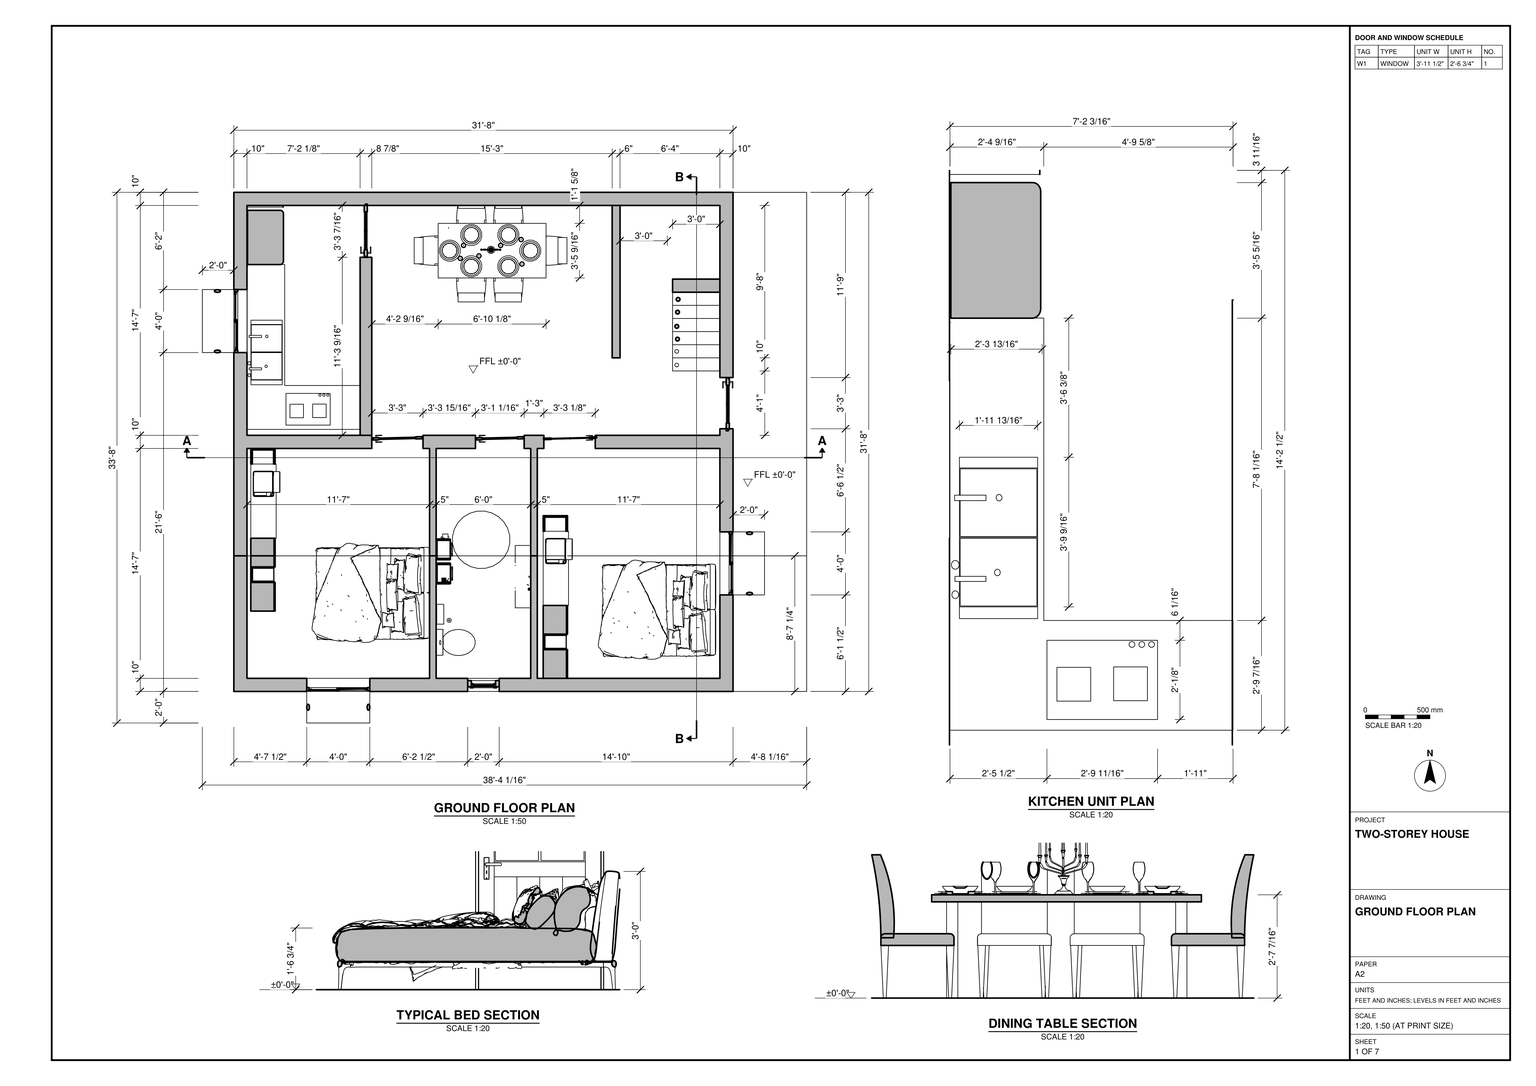
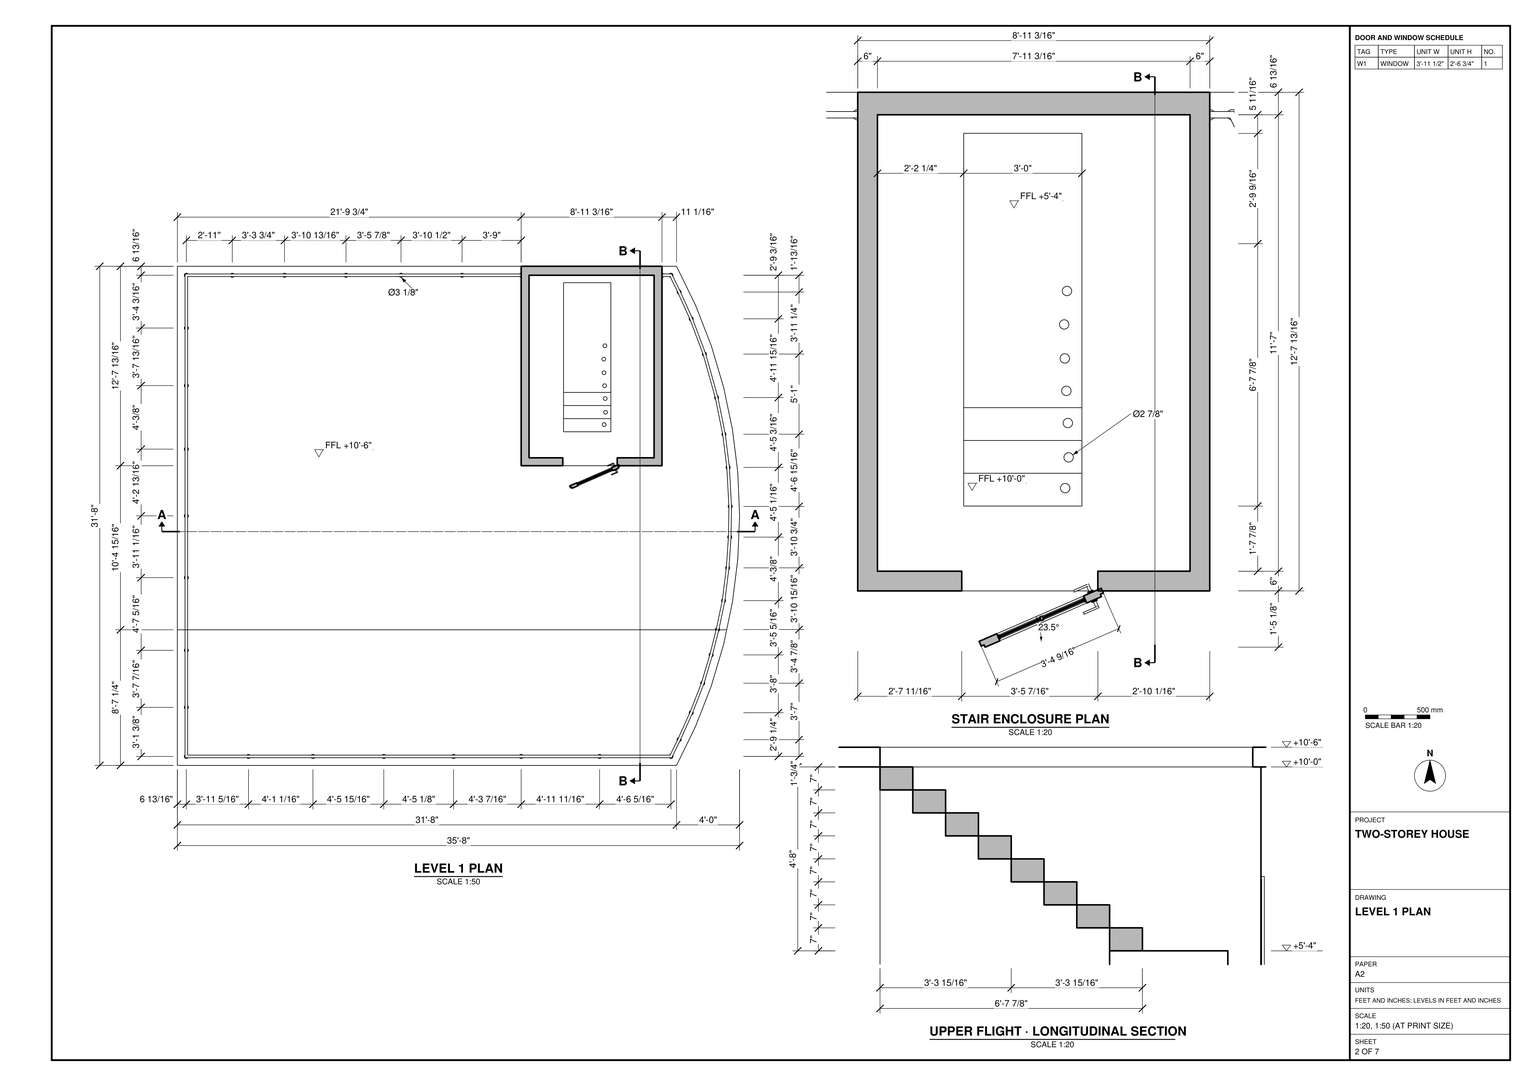
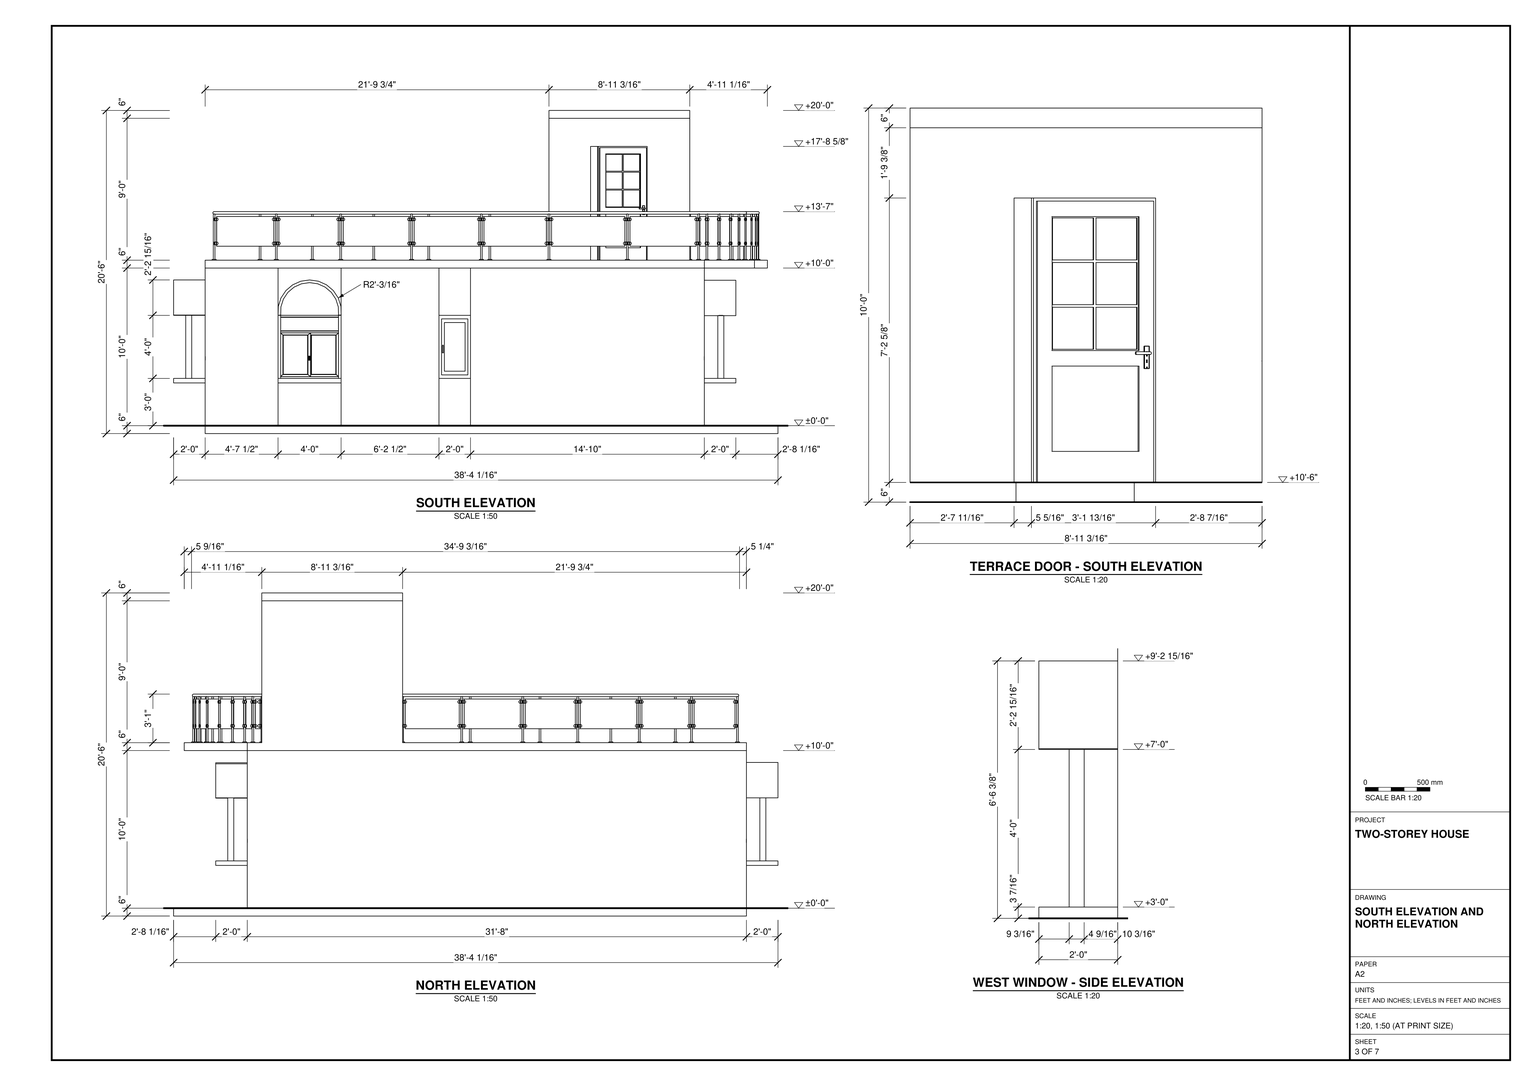
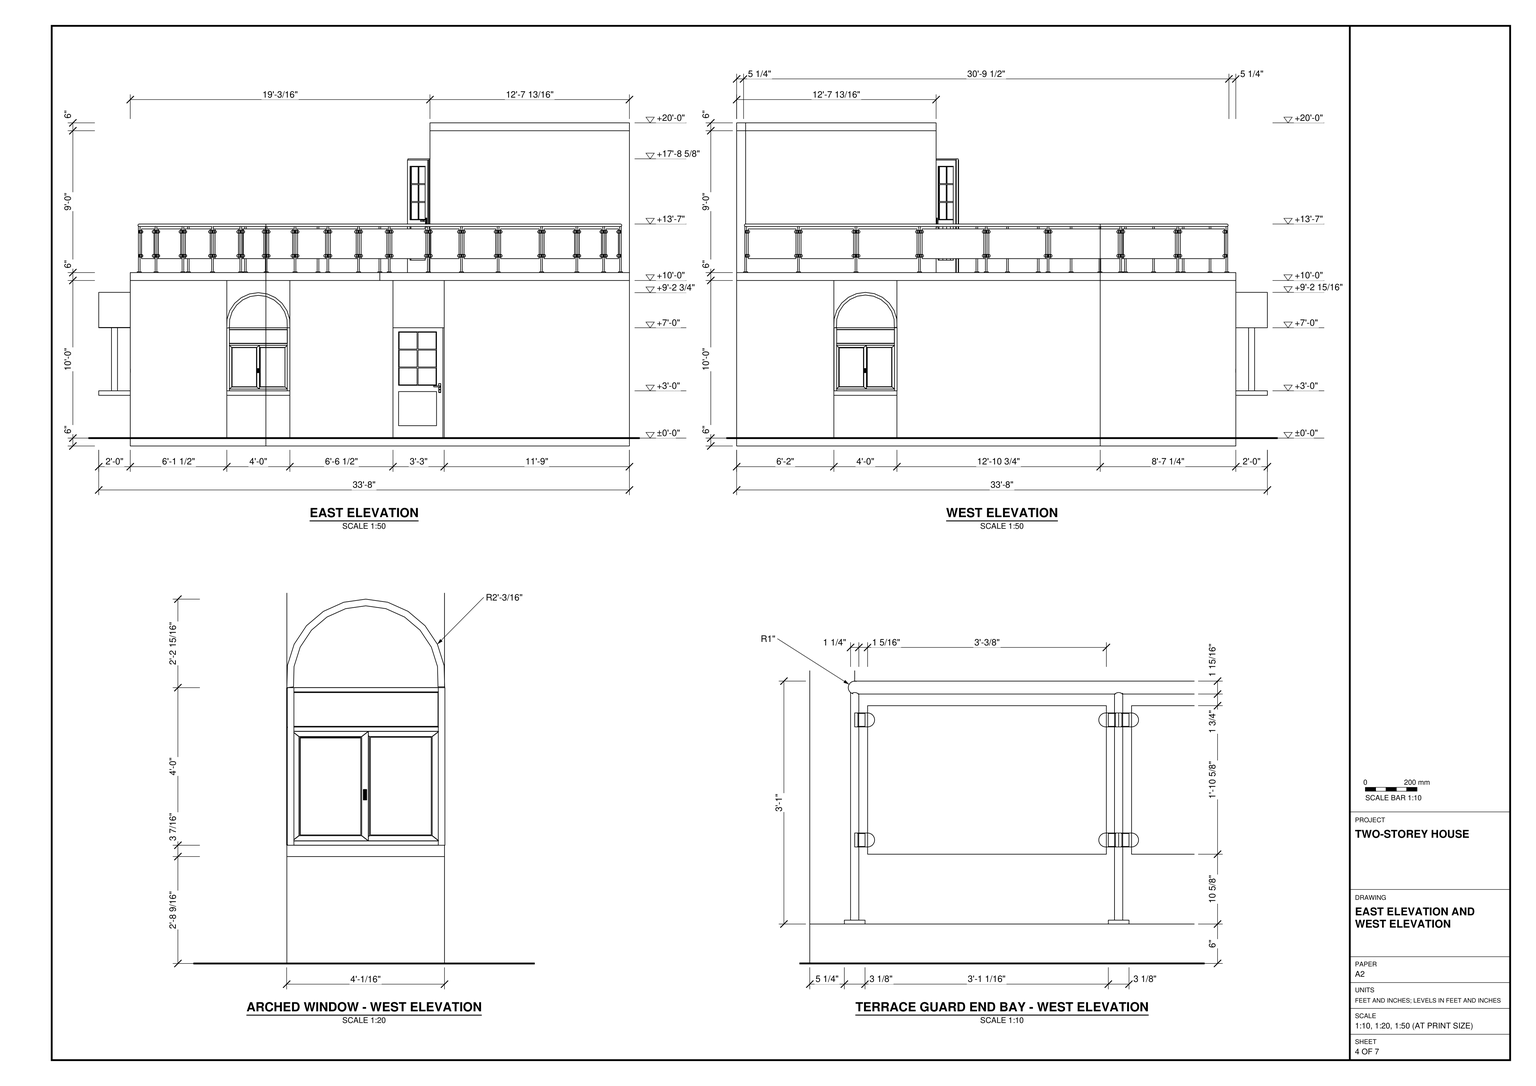
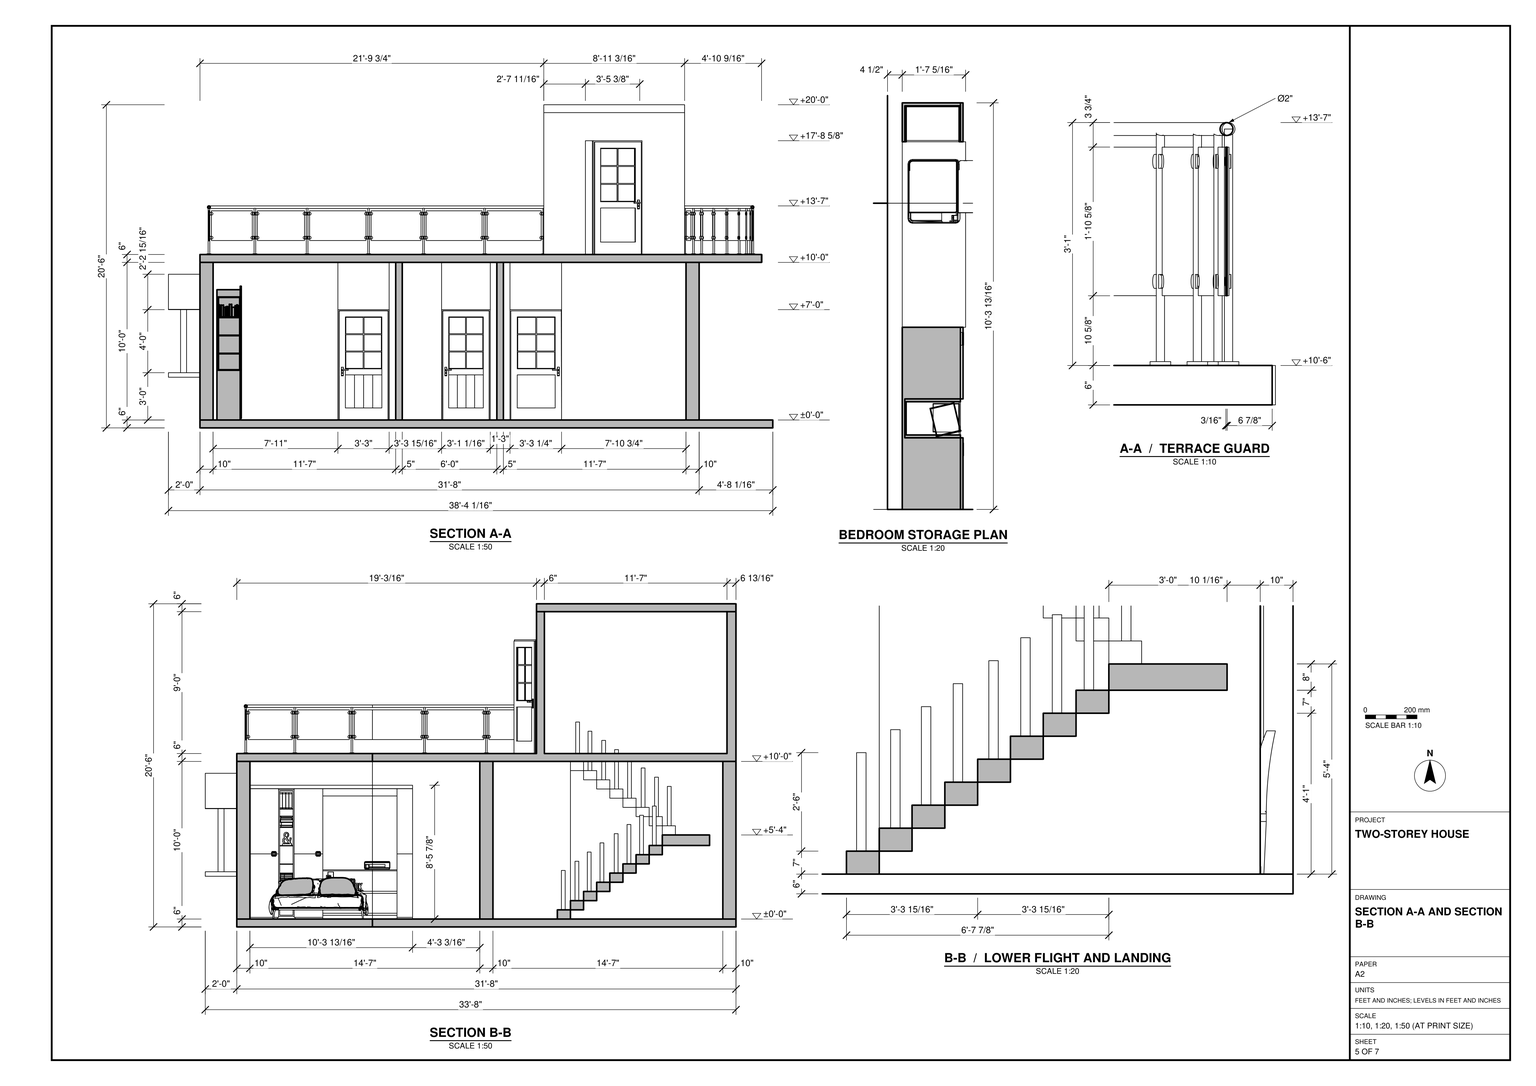
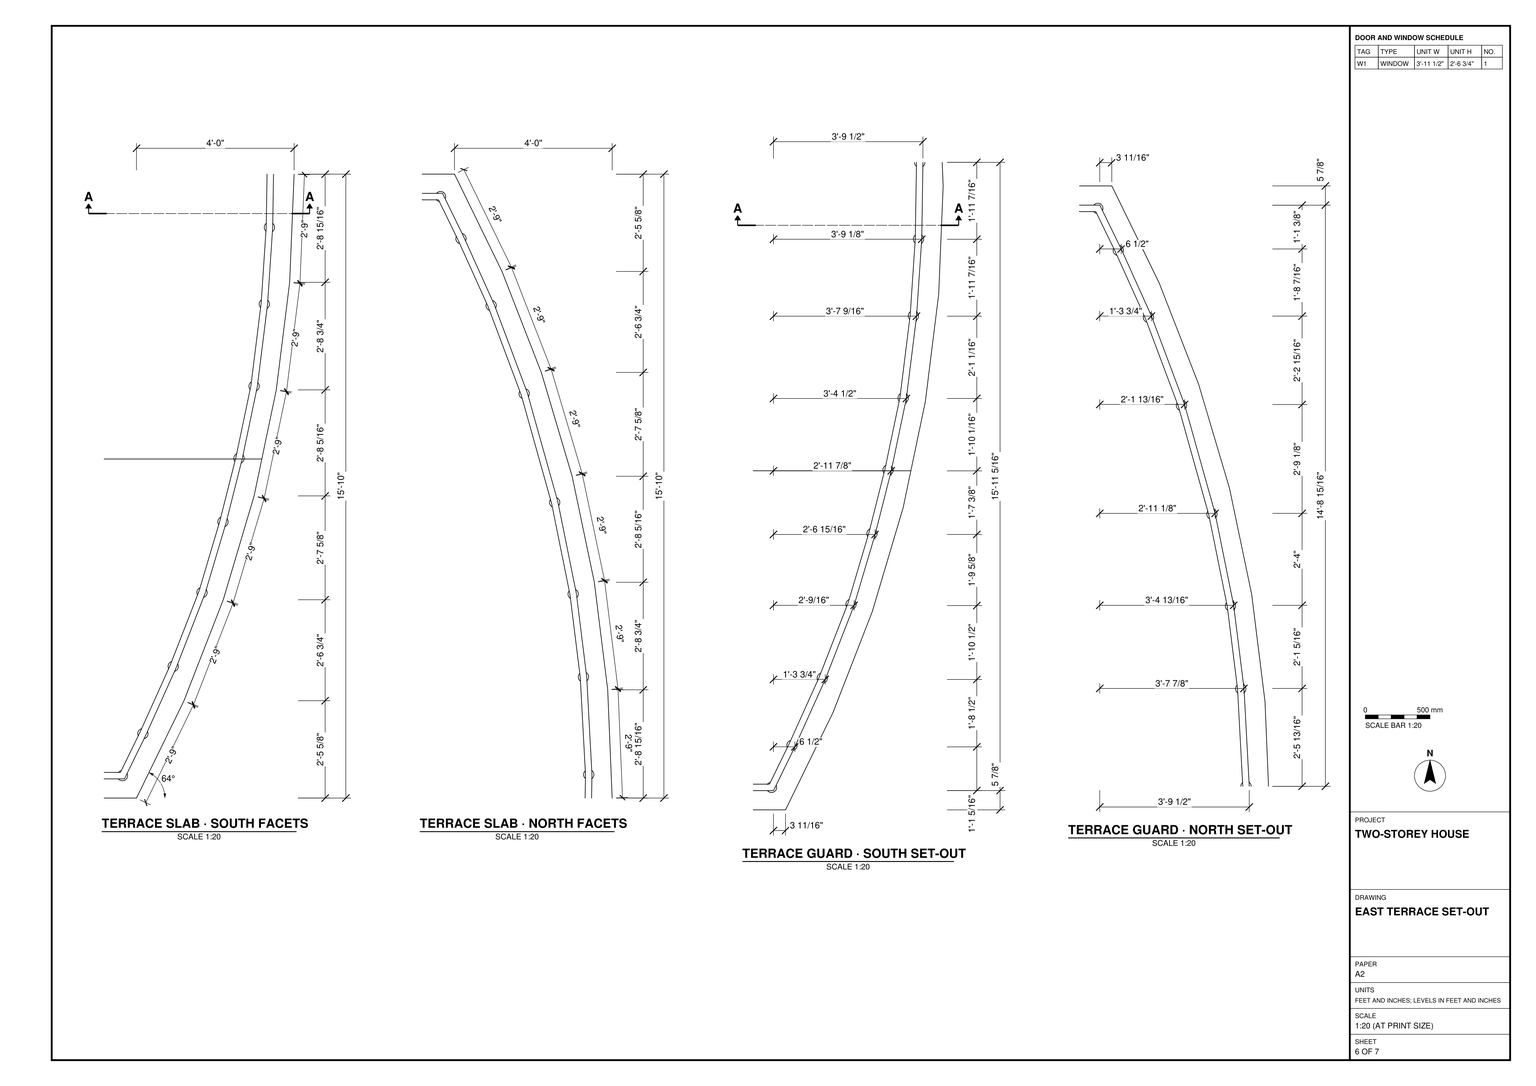
Build the house in SketchUp from task_files/diagram_01.pdf. Work in feet and inches. The overall model extents, including projections, are 38'-4 1/16" east to west, 33'-8" north to south and 20'-6" vertically. Set the ground floor at ±0'-0" and the upper level at +10'-0". Distinguish the upper level from the terrace surface at +10'-6".

Model the ground slab, exterior walls and internal partitions with the thicknesses shown in plan. Place the two bedrooms along the south wall with the bathroom between them. Fit out the bedrooms with the beds and wall-side furniture shown. Place the L-shaped kitchen in the northwest corner, the dining table and chairs beside it, and the stair to the northeast. Form the door and window openings in their drawn positions, including the projecting window heads and sills shown in elevation.

Connect the stair flights at the intermediate landing. Above them, model the flat-roofed stair enclosure and its glazed door onto the terrace. Follow the curved east edge of the terrace slab in plan and carry the railing around the exposed perimeter. Decor and loose items may be any suitable library components.

Keep shell elements such as walls, slabs and roofs, and each furniture or joinery piece, in separate groups or components. Use components for repeated parts. Save one SketchUp model as output_files/two_storey_house_with_a_curved_edge_roof_terrace.skp.

# SketchUp Ruby script. Lengths in inches.
U = 1.inch
M = Sketchup.active_model
def pt(a) = Geom::Point3d.new(a.map { |v| v * U })
def face(e, loops, mat)
  f = e.add_face(loops[0].map { |a| pt(a) })
  loops[1..].each { |l| e.add_face(l.map { |a| pt(a) }).erase! }
  f.material = f.back_material = mat if mat
  f
end
# faces: each face lists its corners as indices into pts; further lists are holes
def faces(e, pts, list, mat = nil) = list.each { |f| face(e, (f[0].is_a?(Array) ? f : [f]).map { |l| l.map { |i| pts[i] } }, mat) }
# xy, xz, yz: faces in a plane at the given z, y or x. An outline is a flat list of corners, or four numbers for a rectangle; further outlines are holes
def ring(l) = l.size == 4 ? [[l[0], l[1]], [l[2], l[1]], [l[2], l[3]], [l[0], l[3]]] : l.each_slice(2).to_a
def flat(e, list, mat, &to3) = list.each { |f| face(e, (f[0].is_a?(Array) ? f : [f]).map { |l| ring(l).map { |u, v| to3.(u, v) } }, mat) }
def xy(e, z, list, mat = nil) = flat(e, list, mat) { |x, y| [x, y, z] }
def xz(e, y, list, mat = nil) = flat(e, list, mat) { |x, z| [x, y, z] }
def yz(e, x, list, mat = nil) = flat(e, list, mat) { |y, z| [x, y, z] }
def lines(e, pts, list) = list.each { |a, b| e.add_line(pt(pts[a]), pt(pts[b])) }
# prism: a flat outline (further loops are holes) pulled along v
def prism(e, loops, v, mat = nil)
  f = face(e, loops, mat); d = Geom::Vector3d.new(v.map { |x| x * U })
  f.pushpull(f.normal.samedirection?(d) ? d.length : -d.length)
end
def box(e, o, s, mat = nil) = prism(e, [[o, [o[0] + s[0], o[1], o[2]], [o[0] + s[0], o[1] + s[1], o[2]], [o[0], o[1] + s[1], o[2]]]], [0, 0, s[2]], mat)
def at(x, y, z, deg = 0) = Geom::Transformation.translation(pt([x, y, z])) * Geom::Transformation.rotation(ORIGIN, Z_AXIS, deg.degrees)
def axes(o, x, y, z) = Geom::Transformation.new([*x, 0, *y, 0, *z, 0, *pt(o).to_a, 1])
def part(name) = M.definitions.add(name)
# library, detail: a bought-in or finely detailed component or shape, given as its bounding box
def library(name, o, s) = part(name).tap { |d| box(d.entities, o, s) }
def detail(e, o, s) = box(e.add_group.entities, o, s)
def put(e, d, t, mat = nil) = e.add_instance(d, t).tap { |i| i.material = mat if mat }
def group(e, t, mat = nil) = e.add_group.tap { |g| g.transformation = t; g.material = mat if mat }.entities
root = M.entities
M.materials.add("Material \#26").color = [4, 4, 4]
M.materials.add("Material \#575").color = [127, 127, 127]
M.materials.add("[Color D02]").color = [255, 229, 153]
M.materials.add("[Color D03]").color = [255, 216, 101]
M.materials.add("[Color E02]").color = [255, 255, 153]
M.materials.add("[Color F02]").color = [204, 255, 153]
M.materials.add("[Color I01]").color = [204, 204, 255]
M.materials.add("[Color_000]").color = [255, 255, 255]
M.materials.add("[Color_004]").color = [142, 142, 142]
M.materials.add("[Color_005]").color = [114, 114, 114]
M.materials.add("[Color_007]").color = [58, 58, 58]
M.materials.add("[Translucent Glass Blue]").color = [100, 149, 237]
M.materials["[Translucent Glass Blue]"].alpha = 0.5
M.materials.add("[Translucent Glass Gray]").color = [0, 0, 0]
M.materials["[Translucent Glass Gray]"].alpha = 0.1
M.materials.add("[Wood_ Floor]").color = [155, 105, 61]
M.materials.add("[Wood_Lumber_ButtJoined]").color = [69, 62, 43]
c1 = library("ear swab",[42.94,49.125,-0.01],[11.74,6.52,7.19])
c2 = library("Window with transom",[0,0,0],[5.2,55.12,70.87])
c3 = library("Deur met glas",[0,0,0],[39.37,7.97,86.61])
c4 = library("Composant\#42",[0,0,0],[23.62,8.27,35.43])
c5 = library("Untitled",[0,-0.39,0],[231.1,401.96,270.47])
c6 = library("Dining Table",[54.55,57.53,0],[71.62,106.71,46.43])
c7 = library("Group\#16",[0,0,0],[13.47,43.07,1.47])
c8 = library("Group\#63",[0,0,0],[5.65,13.74,2.92])
c9 = library("Group\#64",[0,0,0],[6.09,14.19,2.01])
c10 = library("Group\#65",[0,0,0],[2.54,2.54,11.95])
c11 = library("Group\#66",[0,0,0],[2.54,2.54,11.95])
c12 = library("Group\#50",[0,0,0],[19.72,19.72,56.95])
c13 = library("Group\#81",[0,0,0],[3.17,3.17,3.01])
c14 = library("Group\#51",[0,0,-141.09],[175,104.42,354])
c15 = library("Group\#99",[0,0,0],[24,48.09,26.96])
c16 = part("Group\#100")
box(c16.entities,[0,0,0],[48,24,3.44])
c17 = part("Group\#3")
box(c17.entities,[0,0,0],[36,9.99,7])
c18 = library("Group\#104",[0,0,0],[2.875,2.875,30])
c19 = library("Group\#105",[0,0,0],[417.17,369.47,36.98])
c20 = part("Group255\#1")
xz(c20.entities,1200.29,[[724.9375,120,1143.1,126]])
c21 = part("Group259\#1")
xz(c21.entities,1200.29,[[724.9375,0,734.9375,120],[873.9375,0,878.9375,120],[950.9375,0,955.9375,120],[1094.9375,0,1104.9375,36],[1094.9375,84,1104.9375,120]],"[Color E02]")
c22 = part("Group261\#1")
xz(c22.entities,1200.29,[[724.9375,-6,1161,0]],"[Color D03]")
c23 = part("Group2139\#1")
xz(c23.entities,1200.29,[[886.94,28.92,887.95,35.86]])
c24 = part("Group2175\#1")
xz(c24.entities,1200.29,[[889.71,0,890.1,28.92]],"[Wood_Lumber_ButtJoined]")
c25 = part("Group2179\#1")
xz(c25.entities,1200.29,[[890.79,25.29,891.39,26.55]],"[Color_005]")
c26 = part("Group2225\#1")
xz(c26.entities,1200.29,[[895.16,-0.23,931.33,0]])
c27 = part("Group2241\#1")
xz(c27.entities,1200.29,[[755.57,49.61,756.36,99.21]],"[Color_007]")
c28 = part("Group2251\#1")
xz(c28.entities,1200.29,[[755.57,1.26,756.36,49.61]],"[Color_007]")
c29 = part("Group2447\#1")
xz(c29.entities,1200.29,[[737.85,0,755.57,99.21]],"[Color_007]")
c30 = part("Group2455\#1")
xz(c30.entities,1200.29,[[755.57,99.29,756.36,101.87]],"[Color_000]")
c31 = part("Group2495\#1")
xz(c31.entities,1200.29,[[978.15,93.7,978.93,99.21]],"[Color_007]")
c32 = part("Group2681\#1")
xz(c32.entities,1200.29,[[960.43,0,960.43,36.69,962.16,36.69,962.16,21.14,978.15,21.14,978.15,19.57,962.16,19.57,962.16,4.41,978.15,4.41,978.15,2.83,962.16,2.83,962.16,0],[960.43,93.7,978.15,99.21]],"[Color_007]")
c33 = part("Group2683\#1")
xz(c33.entities,1200.29,[[963.06,38.07,962.83,38.1,962.42,38.34,962.18,38.74,962.15,38.98,962.15,42.95,962.18,43.1875,962.34,43.46,965.76,43.46,965.76,43.43,974.03,43.43,974.03,43.46,976.85,43.46,977.14,43.39,977.36,43.17,977.4375,42.875,977.4375,41.61,977.04,39.84,969.5,39.84,969.5,38.07],[969.5,38.07,969.52,39.84],[965.76,43.43,974.03,43.44],[962.3125,43.46,962.3125,43.62,962.32,43.68,962.38,43.79,962.49,43.85,962.55,43.86,976.89,43.86,976.95,43.85,977.05,43.79,977.11,43.68,977.12,43.62,977.12,43.46]],"[Color_000]")
c34 = part("Group2685\#1")
xz(c34.entities,1200.29,[[962.86,37.48,962.78,37.49,962.64,37.57,962.56,37.71,962.55,37.8,962.55,38.26,962.83,38.1,963.06,38.07,977.12,38.07,977.36,38.1,977.4375,38.15,977.4375,37.8,977.43,37.71,977.34,37.57,977.2,37.49,977.12,37.48]],"[Color_000]")
c35 = part("Group2687\#1")
xz(c35.entities,1200.29,[[960.43,36.69,979.72,37.48]],"[Color_000]")
c36 = part("Group2689\#1")
xz(c36.entities,1200.29,[[978.15,99.29,978.93,101.87]],"[Color_000]")
c37 = part("Group2713\#1")
xz(c37.entities,1200.29,[[941.89,85.13,941.89,85.15,941.69,85.15,941.69,85.24,944.33,85.24,944.33,85.15,944.125,85.15,944.125,85.13]])
c38 = part("Group2727\#1")
xz(c38.entities,1200.29,[[939.13,15.53,939.52,24.44]],"[Wood_ Floor]")
c39 = part("Group2741\#1")
xz(c39.entities,1200.29,[[856.47,16.56,856.44,16.57,856.04,16.91,855.92,17.15,855.91,17.21,855.9375,17.43,855.99,17.54,856.04,17.61,856.18,17.65,856.98,17.94,857.07,17.77,857.09,17.71,857.13,17.67,857.22,17.5625,857.4375,17.26,857.52,17.04,857.54,16.99,857.54,16.96,857.53,16.76,857.36,16.63,857.14,16.58],[857.64,17.67,857.52,17.68,857.47,17.7,856.98,17.96,856.95,18.01,856.82,18.23,856.74,18.42,856.68,18.58,856.67,18.64,856.61,19.1,856.65,19.38,856.66,19.43,856.72,19.5,856.91,19.83,857.07,19.87,857.24,20.06,857.51,20.29,857.76,20.47,857.84,20.71,857.88,20.79,857.95,20.85,858.23,20.95,858.4375,20.97,858.48,21,858.57,21.26,858.64,21.37,858.66,21.4375,858.86,21.53,858.89,21.59,859.18,21.78,859.36,21.83,859.49,21.93,859.63,22.1875,859.87,22.39,860.21,22.59,860.22,22.59,860.28,22.65,860.25,22.58,860.24,22.58,860.11,22.19,860.1,22.14,859.83,21.55,859.74,21.27,859.53,20.97,859.49,20.93,859.45,20.9,859.45,20.4,859.29,20.39,859.22,20.22,859.17,20.12,859.16,19.77,859.125,19.73,858.91,19.16,858.87,19.1,858.85,19.04,858.6875,18.89,858.63,18.64,858.5,18.44,858.3125,18.1,858.16,17.92,858.0625,17.86,857.83,17.73,857.7,17.68],[860.41,22.91,860.64,23.3,860.79,23.58,860.93,23.8,861.18,24.21,861.44,24.6875,861.5,24.78,862.15,25.52,862.32,25.73,862.72,26.125,862.73,26.125,862.73,26.13,863.6,26.67,863.92,26.64,863.92,26.74,863.86,26.86,864.09,27.03,864.11,27.07,864.13,27.14,864.1,27.46,864.06,27.55,864.08,27.67,864.17,27.92,864.19,27.97,864.67,28.58,864.88,28.83,864.98,29.08,865.07,29.41,865.24,29.78,865.33,29.89,865.35,30.11,865.45,30.41,865.57,30.58,865.65,30.8125,865.65,31.11,865.66,31.16,865.6875,31.25,865.93,31.89,865.96,32.07,866.05,32.16,866.26,32.29,866.42,32.35,866.55,32.39,866.59,32.375,866.7,32.37,867.05,32.3,867.1,32.32,867.11,32.44,867.11,32.76,867.26,32.86,867.31,32.89,867.39,32.68,867.45,32.6,867.23,32.29,867.22,32.02,867.23,32.01,867.29,31.97,867.22,31.83,867.21,31.625,866.98,31.47,866.93,31.47,866.62,31.49,866.59,31.36,866.63,31.1,866.5,30.87,866.45,30.76,866.4375,30.42,866.46,30.28,866.36,30.04,866.32,29.93,866.19,29.73,865.96,29.38,865.82,29.25,865.75,29.18,865.57,29.09,865.47,28.94,865.28,28.72,865.09,28.46,865.05,28.5,864.67,28.01,864.4,27.73,864.42,27.51,864.4,27.27,864.37,27.04,864.38,26.84,864.31,26.3,864.22,26.33,864.125,26.15,864.45,25.63,864.45,25.61,864.42,25.5625,864.12,25.15,863.71,24.61,863.65,24.53,863.18,24.39,863.08,24.43,862.76,24.73,862.63,24.78,862.52,24.69,862.13,24.39,861.8,24.36,861.33,23.9,861.1,23.66,861.04,23.52,860.87,23.34,860.75,23.25]])
c40 = part("Group2753\#1")
xy(c40.entities,8.38,[[868.6,1200.29,868.61,1200.29,868.61,1200.29],[868.61,1200.29,868.62,1200.29,868.61,1200.29]],"Material \#26")
xz(c40.entities,1200.29,[[862.63,8.38,862.45,8.43,862.43,8.4375,862.45,8.43,862.66,8.38],[868.61,8.38,868.61,8.38,868.79,8.42,868.62,8.38]],"Material \#26")
c41 = part("Group2755\#1")
xz(c41.entities,1200.29,[[788.39,6.89,788.27,6.93,788.15,8.56,788.15,8.5625,788.375,8.76,788.38,8.77,788.51,8.82,789.05,8.68,789.16,8.5625,789.16,8.56,788.74,7.01],[872.375,6.89,872.02,7.01,871.53,8.4,871.53,8.41,871.61,8.56,871.61,8.5625,871.83,8.76,871.83,8.77,871.97,8.82,872.61,8.5625,872.61,8.56,872.69,8.41,872.69,8.4,872.64,7.12,872.63,7.12,872.54,6.97,872.49,6.93]],"Material \#575")
c42 = part("Group2767\#1")
xz(c42.entities,1200.29,[[880.52,71.11,880.4375,71.23,880.45,71.24,880.53,71.12]])
c43 = part("Group2871\#1")
xz(c43.entities,1200.29,[[886.78,67.95,886.78,67.96,886.77,67.97,886.77,67.98,886.76,68,886.76,68.02,886.77,68.03,886.77,68.0625,886.78,68.07],[886.78,67.95,886.79,68.07],[886.79,67.95,886.79,68.07,886.79,68.0625,886.8,68.05,886.8,68.02,886.81,68,886.8,67.99,886.8,67.97,886.79,67.96]])
c44 = part("Group2931\#1")
xz(c44.entities,1200.29,[[886.54,68.83,886.54,68.84,886.53,68.85,886.53,68.86,886.52,68.88,886.52,68.9375,886.53,68.96,886.53,68.97,886.54,68.9],[886.54,68.83,886.54,68.9,886.53,68.97,886.54,68.97,886.56,68.83],[886.56,68.83,886.54,68.97,886.55,68.97,886.56,68.95,886.5625,68.93,886.57,68.92,886.57,68.86,886.56,68.84]])
c45 = part("Group3049\#1")
xz(c45.entities,1200.29,[[884.48,66.66,884.48,66.67,884.51,66.68,884.52,66.68,884.52,66.67]])
c46 = part("Group3063\#1")
xz(c46.entities,1200.29,[[886.35,70.0625,886.26,70.125,886.27,70.16,886.33,70.12,886.35,70.1]])
c47 = part("Group3285\#1")
xz(c47.entities,1200.29,[[1101.97,70.66,1101.95,70.69,1101.95,71.97,1101.97,71.99,1104.19,71.99,1104.21,71.97,1104.21,70.69,1104.19,70.66]],"[Color F02]")
c48 = part("Group3287\#1")
xz(c48.entities,1200.29,[[1101.97,35.97,1101.95,36,1101.95,37.28,1101.97,37.3,1104.19,37.3,1104.21,37.28,1104.21,36,1104.19,35.97]],"[Color F02]")
c49 = part("Group3289\#1")
xz(c49.entities,1200.29,[[1101.97,82.67,1101.95,82.69,1101.95,83.97,1101.97,84,1104.19,84,1104.21,83.97,1104.21,82.69,1104.19,82.67]],"[Color F02]")
c50 = part("Group3299\#1")
xz(c50.entities,1200.29,[[1103.02,72.21,1103.14,82.45]],"[Translucent Glass Gray]")
c51 = part("Group3315\#1")
xz(c51.entities,1200.29,[[1102.99,71.99,1103.17,72.21],[1102.99,82.45,1103.17,82.67]],"[Color F02]")
c52 = part("Group3323\#1")
xz(c52.entities,1200.29,[[1102.8,39.12,1102.91,68.84]],"[Translucent Glass Gray]")
c53 = part("Group3325\#1")
xz(c53.entities,1200.29,[[1102.76,38.91,1102.94,39.12],[1102.76,68.84,1102.94,69.06]],"[Color F02]")
c54 = part("Group3327\#1")
xz(c54.entities,1200.29,[[1102.42,37.3,1102.4,37.33,1102.4,38.88,1102.42,38.91,1103.28,38.91,1103.31,38.88,1103.31,37.33,1103.28,37.3]],"[Color F02]")
c55 = part("Group3329\#1")
xz(c55.entities,1200.29,[[1102.42,69.06,1102.4,69.08,1102.4,70.63,1102.42,70.66,1103.28,70.66,1103.31,70.63,1103.31,69.08,1103.28,69.06]],"[Color F02]")
c56 = part("Group3661\#1")
xz(c56.entities,1200.29,[[1104.9375,107.875,1128.9375,109.91]],"[Color F02]")
c57 = part("Group3671\#1")
xz(c57.entities,1200.29,[[1104.9375,32.56,1128.9375,36]],"[Color F02]")
c58 = part("Group3741\#1")
xz(c58.entities,1200.29,[[1134.62,126,1135.58,126.59],[1135.58,126,1136.75,126.59],[1136.75,126,1137.71,126.59],[[1135.58,126.59,1135.58,161.17,1135.6,161.15,1135.84,161.05,1136.11,161.02,1136.37,161.05,1136.61,161.15,1136.75,161.25,1136.75,126.59],[1135.72,156.02,1136.01,156.02,1136.01,156.09,1136.21,156.09,1136.21,156.02,1136.49,156.02,1136.49,158.14,1136.21,158.14,1136.21,158.0625,1136.01,158.0625,1136.01,158.14,1135.72,158.14],[1136.21,137.73,1136.49,139.86]],[731.68,136.63,731.875,159.24],
  [1135.72,137.73,1136.01,139.86],[1136.01,137.8125,1136.21,139.78],[1136.01,156.09,1136.21,158.0625],[731.78,161.02,731.52,161.05,731.29,161.15,731.08,161.3,730.93,161.51,730.83,161.75,730.79,162,730.83,162.25,730.93,162.49,731.08,162.7,731.29,162.85,731.52,162.95,731.78,162.98,732.03,162.95,732.27,162.85,732.47,162.7,732.63,162.49,732.73,162.25,732.76,162,732.73,161.75,732.63,161.51,732.47,161.3,732.27,161.15,732.03,161.05],[1135.58,161.17,1135.39,161.3,1135.23,161.51,1135.125,161.75,1135.09,162,1135.125,162.25,1135.23,162.49,1135.39,162.7,1135.6,162.85,1135.84,162.95,1136.11,162.98,1136.37,162.95,1136.61,162.85,1136.82,162.7,1136.99,162.49,1137.09,162.25,1137.1,162.17,1137.12,162,1137.1,161.83,1137.09,161.75,1136.99,161.51,1136.82,161.3,1136.75,161.25,1136.75,162,1135.58,162]])
c59 = part("Group254\#1")
xz(c59.entities,1200.29,[[866.98,8.64,866.64,8.65,866.625,8.66,866.49,8.73,866.48,8.73,866.39,8.66,866.3125,8.6875,866.25,8.74,866.26,8.8,866.3,8.87,866.23,8.85,866.2,8.87,866.1,8.95,865.91,9.22,865.87,9.28,865.79,9.4375,865.64,9.75,865.92,10.27,866.03,10.48,866.03,10.53,866.06,10.67,866.11,10.85,866.14,11.14,866.14,11.19,866.15,11.34,866.14,11.41,866.23,12.22,866.24,12.64,866.26,13.17,866.26,13.61,866.25,14.23,866.22,14.88,866.22,15.02,866.18,15.35,866.17,15.5,866.14,15.71,866.12,15.8,866.07,16.05,866.01,16.31,865.99,16.39,865.9375,16.54,865.89,16.71,865.87,16.76,865.74,17.01,865.67,17.14,865.58,17.29,865.47,17.41,866.45,24.05,866.58,24.8,867.67,31.02,867.7,31.15,868.04,32.57,868.08,32.68,868.55,33.86,869.04,34.85,869.24,35.23,869.28,35.3,869.32,35.375,869.53,35.68,869.65,35.78,869.72,35.76,869.68,35.82,869.68,35.89,869.74,35.94,869.82,35.97,869.91,35.9,869.91,35.91,870.02,36.01,870.03,36.01,870.29,36.07,870.36,36.08,870.84,36.07,871.6,36.04,871.75,36.03,872.51,35.94,872.98,35.84,873.03,35.83,873.04,35.83,873.29,35.73,873.3,35.73,873.38,35.65,873.39,35.61,873.49,35.65,873.5625,35.6,873.61,35.53,873.56,35.43,873.59,35.42,873.65,35.3,873.73,34.97,873.81,34.38,873.81,34.37,873.9,33.41,873.9,33.25,873.94,32.05,873.93,31.92,873.85,30.49,873.77,29.6,873,20.35,872.54,14.23,872.5,13.64,872.48,13.51,872.34,12.1,872.15,10.94,872.125,10.81,872.12,10.78,872.11,10.75,871.92,9.95,871.89,9.83,871.74,9.28,871.62,8.97,871.51,8.85,871.54,8.75,871.48,8.69,871.39,8.65,871.3,8.7,871.14,8.65,867.54,8.64],[865.64,9.75,865.57,9.89,865.5625,9.91,865.53,10,865.19,10.92,865.18,11.04,864.95,12.25,864.95,12.39,864.99,13.85,865.01,14,865.2,15.59,865.29,16.19,865.47,17.41,865.58,17.29,865.67,17.14,865.74,17.01,865.87,16.76,865.89,16.71,865.9375,16.54,865.99,16.39,866.01,16.31,866.07,16.05,866.12,15.8,866.14,15.71,866.17,15.5,866.18,15.35,866.22,15.02,866.22,14.88,866.25,14.23,866.26,13.61,866.26,13.17,866.24,12.64,866.23,12.22,866.14,11.41,866.15,11.34,866.14,11.19,866.14,11.14,866.11,10.85,866.06,10.67,866.03,10.53,866.03,10.48,865.92,10.27]])
# 772 loose lines left out
put(c59.entities,c20,at(0,0,0))
put(c59.entities,c21,at(0,0,0))
put(c59.entities,c22,at(0,0,0))
put(c59.entities,c23,at(0,0,0))
put(c59.entities,c24,at(0,0,0))
put(c59.entities,c25,at(0,0,0))
put(c59.entities,c26,at(0,0,0))
put(c59.entities,c27,at(0,0,0))
put(c59.entities,c28,at(0,0,0))
put(c59.entities,c29,at(0,0,0))
put(c59.entities,c30,at(0,0,0))
put(c59.entities,c31,at(0,0,0))
put(c59.entities,c32,at(0,0,0))
put(c59.entities,c33,at(0,0,0))
put(c59.entities,c34,at(0,0,0))
put(c59.entities,c35,at(0,0,0))
put(c59.entities,c36,at(0,0,0))
put(c59.entities,c37,at(0,0,0))
put(c59.entities,c38,at(0,0,0))
put(c59.entities,c39,at(0,0,0))
put(c59.entities,c40,at(0,0,0))
put(c59.entities,c41,at(0,0,0))
put(c59.entities,c42,at(0,0,0))
put(c59.entities,c43,at(0,0,0))
put(c59.entities,c44,at(0,0,0))
put(c59.entities,c45,at(0,0,0))
put(c59.entities,c46,at(0,0,0))
put(c59.entities,c47,at(0,0,0))
put(c59.entities,c48,at(0,0,0))
put(c59.entities,c49,at(0,0,0))
put(c59.entities,c50,at(0,0,0))
put(c59.entities,c51,at(0,0,0))
put(c59.entities,c52,at(0,0,0))
put(c59.entities,c53,at(0,0,0))
put(c59.entities,c54,at(0,0,0))
put(c59.entities,c55,at(0,0,0))
put(c59.entities,c56,at(0,0,0))
put(c59.entities,c57,at(0,0,0))
put(c59.entities,c58,at(0,0,0))
xy(root,0,[[312,278,318,394]])
xy(root,0,[[120.125,219,129,354.55]],"[Color D02]")
xy(root,84,[[394,224,404,263]])
xy(root,86.61,[[120.125,354.55,124.02,394],[124.02,354.55,129,394]],"[Color D02]")
xy(root,120,[[312,278,318,394]])
xy(root,120,[[120.125,219,129,394],[394,224,404,263]],"[Color D02]")
xy(root,120,[[[24,24,404,24,418.46,53.65,430.42,84.39,439.8125,116.02,446.57,148.3,450.64,181.04,452,214,450.64,246.96,446.57,279.7,439.8125,311.98,430.42,343.61,418.46,374.35,404,404,24,404],[312,278,312,394,318,394,318,391.5,354,391.5,354,278],[120.125,219,129,394],[394,224,404,263]]],"[Color F02]")
xy(root,126,[[24,24,404,24,418.46,53.65,430.42,84.39,439.8125,116.02,446.57,148.3,450.64,181.04,452,214,450.64,246.96,446.57,279.7,439.8125,311.98,430.42,343.61,418.46,374.35,404,404,392.93,404,392.93,397.16,399.73,397.16,412.1875,371.61,423.95,341.39,433.18,310.31,439.82,278.57,443.82,246.4,445.16,214,443.82,181.6,439.82,149.43,433.18,117.69,423.95,86.61,412.1875,56.39,399.73,30.84,30.84,30.84,30.84,397.16,285.74,397.16,285.74,404,24,404],[30.84,30.84,399.73,30.84,412.1875,56.39,423.95,86.61,433.18,117.69,439.82,149.43,443.82,181.6,445.16,214,443.82,246.4,439.82,278.57,433.18,310.31,423.95,341.39,412.1875,371.61,399.73,397.16,392.93,397.16,392.93,252.16,285.74,252.16,285.74,397.16,30.84,397.16],[[317.41,252.16,358.85,252.16,358.85,258.16,386.93,258.16,386.93,397.16,291.74,397.16,291.74,258.16,317.41,258.16],[318,278,354,391.5]]],"[Color F02]")
xy(root,212.61,[[317.41,252.16,358.85,258.16]],"[Color F02]")
xy(root,234,[[[285.74,252.16,392.93,404],[291.74,258.16,386.93,397.16]]],"[Color F02]")
xz(root,24,[[24,120,404,126]],"[Color F02]")
xz(root,25.77,[[81.42,72.24,125.51,82.48]],"[Translucent Glass Blue]")
xz(root,219,[[120.125,0,129,120]],"[Color D02]")
xz(root,224,[[394,84,404,120]])
xz(root,252.16,[[285.74,126,317.41,126,317.41,212.61,358.85,212.61,358.85,126,392.93,126,392.93,234,285.74,234]],"[Color F02]")
xz(root,258.16,[[291.74,126,291.74,234,386.93,234,386.93,126,358.85,126,358.85,212.61,317.41,212.61,317.41,126]],"[Color F02]")
xz(root,263,[[394,84,404,120]])
xz(root,278,[[312,0,318,120]])
xz(root,278,[[318,120,354,126]],"[Color F02]")
xz(root,354.55,[[120.125,0,129,86.61]],"[Color D02]")
xz(root,391.5,[[318,120,354,126]],"[Color F02]")
xz(root,394,[[312,0,318,120]])
xz(root,394,[[120.125,86.61,129,120]],"[Color D02]")
xz(root,397.16,[[291.74,126,386.93,234]],"[Color F02]")
xz(root,404,[[24,120,24,126,285.74,126,285.74,234,392.93,234,392.93,126,404,126,404,120]],"[Color F02]")
yz(root,24,[[24,120,404,126]],"[Color F02]")
yz(root,25.77,[[283.99,72.24,328.08,82.48]],"[Translucent Glass Blue]")
yz(root,25.99,[[286.05,39.15,304.56,68.875]],"[Translucent Glass Blue]")
yz(root,120.125,[[219,0,219,120,394,120,394,86.61,354.55,86.61,354.55,0]],"[Color D02]")
yz(root,129,[[219,0,354.55,0,354.55,86.61,394,86.61,394,120,219,120]],"[Color D02]")
yz(root,285.74,[[252.16,126,397.16,234],[397.16,126,404,234]],"[Color F02]")
yz(root,291.74,[[258.16,126,397.16,234]],"[Color F02]")
yz(root,312,[[278,0,394,120]])
yz(root,317.41,[[252.16,126,258.16,212.61]],"[Color F02]")
yz(root,318,[[278,120,391.5,126]],"[Color F02]")
yz(root,318,[[278,0,394,120]],"[Color I01]")
yz(root,354,[[278,120,391.5,126]],"[Color F02]")
yz(root,358.85,[[252.16,126,258.16,212.61]],"[Color F02]")
yz(root,386.93,[[258.16,126,397.16,234]],"[Color F02]")
yz(root,392.93,[[252.16,126,404,234]],"[Color F02]")
yz(root,394,[[224,84,263,120]],"[Color D03]")
yz(root,400.6,[[228.69,40.55,242.32,53.35],[243.13,40.55,256.76,53.35],[228.69,54.13,242.32,66.97],[243.13,54.13,256.76,66.97],[228.69,67.76,242.32,80.55],
  [243.13,67.76,256.76,80.55]],"[Translucent Glass Blue]")
yz(root,402.01,[[123.01,39.12,141.52,68.84]])
yz(root,402.23,[[99.49,72.21,143.58,82.45]],"[Translucent Glass Blue]")
yz(root,402.91,[[101.55,39.12,120.06,68.84]],"[Translucent Glass Blue]")
yz(root,404,[[224,84,263,120]],"[Color E02]")
# 3 loose lines left out
p = [[83.48,24.93,68.875],[83.48,24.75,38.94],[102.21,24.75,38.94],[102.21,24.93,68.875],[104.71,25.65,68.875],[104.71,25.65,38.94],
  [123.45,25.99,38.94],[123.45,25.99,68.875],[402.35,141.75,68.84],[402.01,123.01,68.84],[402.01,123.01,39.12],[402.01,123.01,38.91],
  [402.35,141.75,38.91],[25.15,325.9,39.15],[25.09,307.51,39.15],[25.09,307.51,68.66],[25.15,325.9,68.66],[418.46,53.65,126],
  [404,24,126],[404,24,120],[418.46,53.65,120],[430.42,84.39,126],[430.42,84.39,120],[439.8125,116.02,126],
  [439.8125,116.02,120],[446.57,148.3,126],[446.57,148.3,120],[450.64,181.04,126],[450.64,181.04,120],[452,214,126],
  [452,214,120],[450.64,246.96,126],[450.64,246.96,120],[446.57,279.7,126],[446.57,279.7,120],[439.8125,311.98,126],
  [439.8125,311.98,120],[430.42,343.61,126],[430.42,343.61,120],[418.46,374.35,126],[418.46,374.35,120],[404,404,126],
  [404,404,120]]
faces(root,p,[[0,1,2,3],[4,5,6,7],[8,9,10,11,12],[13,14,15,16]],"[Translucent Glass Blue]")
faces(root,p,[[17,18,19,20],[21,17,20,22],[23,21,22,24],[25,23,24,26],[27,25,26,28],[29,27,28,30],[31,29,30,32],[33,31,32,34],
  [35,33,34,36],[37,35,36,38],[39,37,38,40],[41,39,40,42]],"[Color F02]")
detail(root,[414.27,97.48,36],[4.58,2.02,48])
detail(root,[414.27,143.5,36],[4.58,2.02,48])
detail(root,[79.5,9.71,36],[2.02,4.58,48])
detail(root,[125.48,9.71,36],[2.02,4.58,48])
detail(root,[9.22,327.85,36],[4.58,2.02,48])
detail(root,[9.22,281.875,36],[4.58,2.02,48])
put(root,c1,axes([160.79,82.61,43.07],[0.5,0,0],[0,0.5,0],[0,0,0.5]))
put(root,c2,axes([401.01,97.5,35.97],[0.57576,0,0],[0,0.87217,0],[0,0,0.67776]),"[Color F02]")
put(root,c2,axes([79.43,26.99,36],[0,-0.57576,0],[0.87217,0,0],[0,0,0.67776]))
put(root,c2,axes([26.99,330.07,36],[-0.57576,0,0],[0,-0.87217,0],[0,0,0.67776]))
put(root,c3,axes([396.03,263,0],[0,-1.03,0],[1,0,0],[0,0,1]),"[Translucent Glass Blue]")
put(root,c3,axes([300.18,219.08,0],[-1.02969,-0.02519,0],[0.01125,-0.46005,0],[0,0,0.96982]))
put(root,c3,axes([208.07,213.59,0],[0.93928,0.02298,0],[-0.0166,0.67878,0],[0,0,0.96982]))
put(root,c3,axes([129.13,213.54,0],[0.99057,0.02423,0],[-0.01676,0.68498,0],[0,0,0.96982]))
put(root,c4,axes([202,24,36],[1.016,0,0],[0,1,0],[0,0,1.35467]),"[Translucent Glass Blue]")
put(root,c5,axes([34,223.52,0],[0.37359,0,0],[0,0.42453,0],[0,0,0.44367]))
put(root,c3,axes([128.4,354.48,0],[0,1.03,0],[-1,0,0],[0,0,1]),"[Translucent Glass Blue]")
put(root,c6,axes([98.57,458.09,0],[0,-1.09,0],[1.09,0,0],[0,0,1.09]))
put(root,c3,axes([358.77,255.54,126],[-0.94457,-0.41071,0],[0.39875,-0.91706,0],[0,0,1]),"[Translucent Glass Blue]")
g1 = group(root,at(24,24,0),"[Color E02]")
xy(g1,0,[[0,0,0,306,10,306,10,195,105,195,105,185,10,185,10,10,149,10,149,185,144,185,144,195,183.9375,195,183.9375,185,154,185,154,10,370,10,370,185,275.27,185,275.27,195,370,195,370,200,380,200,380,0],[226,10,231,185],[221,185,236,195],[370,239,370,370,10,370,10,306,0,306,0,380,380,380,380,239]])
xy(g1,36,[[55.5,0,103.5,10],[178,0,202,10],[370,73.5,380,121.5],[0,258,10,306]])
xy(g1,84,[[55.5,0,103.5,10],[178,0,202,10],[370,73.5,380,121.5],[183.9375,185,221,195],[236,185,275,195],
  [0,258,10,306]])
xy(g1,120,[[0,0,55.5,0,55.5,10,10,10,10,185,105,185,105,195,10,195,10,258,0,258],[55.5,0,103.5,10],[103.5,0,178,0,178,10,154,10,154,185,183.9375,185,183.9375,195,144,195,144,185,149,185,149,10,103.5,10],[178,0,202,10],[202,0,380,0,380,73.5,370,73.5,370,10,231,10,231,185,370,185,370,121.5,380,121.5,380,200,370,200,370,195,221,195,221,185,226,185,226,10,202,10],
  [370,73.5,380,121.5],[105,185,144,195],[183.9375,185,221,195],[370,239,380,239,380,380,0,380,0,306,10,306,10,370,370,370],[0,258,10,306]])
xz(g1,0,[[0,0,55.5,120],[55.5,0,103.5,36],[103.5,0,178,120],[178,0,202,36],[202,0,380,120],
  [55.5,84,103.5,120],[178,84,202,120]])
xz(g1,10,[[10,0,55.5,120],[55.5,0,103.5,36],[103.5,0,149,120],[154,0,178,120],[178,0,202,36],
  [202,0,226,120],[231,0,370,120],[55.5,84,103.5,120],[178,84,202,120]])
xz(g1,73.5,[[370,36,380,84],[370,84,380,120]])
xz(g1,121.5,[[370,36,380,84],[370,84,380,120]])
xz(g1,185,[[10,0,105,120],[144,0,149,120],[154,0,183.9375,120],[221,0,226,120],[231,0,236,120],
  [275.27,0,275.27,120,236,120,236,84,275,84],[275.27,0,370,120],[105,84,144,120],[183.9375,84,221,120]])
xz(g1,195,[[10,0,105,120],[144,0,183.9375,120],[221,0,221,120,370,120,370,0,275.27,0,275,84,236,84,236,0],[105,84,144,120],[183.9375,84,221,120]])
xz(g1,200,[[370,0,380,120]])
xz(g1,239,[[370,0,380,120]])
xz(g1,258,[[0,36,10,84],[0,84,10,120]])
xz(g1,306,[[0,0,10,36],[0,36,10,84],[0,84,10,120]])
xz(g1,370,[[10,0,370,120]])
xz(g1,380,[[0,0,380,120]])
yz(g1,0,[[0,0,258,120],[258,0,306,36],[306,0,380,120],[258,84,306,120]])
yz(g1,10,[[10,0,185,120],[195,0,258,120],[258,0,306,36],[306,0,370,120],[258,84,306,120]])
yz(g1,55.5,[[0,36,10,84],[0,84,10,120]])
yz(g1,103.5,[[0,36,10,84],[0,84,10,120]])
yz(g1,105,[[185,0,195,36],[185,36,195,120]])
yz(g1,144,[[185,0,195,36],[185,36,195,120]])
yz(g1,149,[[10,0,185,120]])
yz(g1,154,[[10,0,185,120]])
yz(g1,178,[[0,36,10,84],[0,84,10,120]])
yz(g1,183.9375,[[185,0,195,36],[185,36,195,84],[185,84,195,120]])
yz(g1,202,[[0,36,10,84],[0,84,10,120]])
yz(g1,221,[[185,0,195,36],[185,36,195,84],[185,84,195,120]])
yz(g1,226,[[10,0,185,120]])
yz(g1,231,[[10,0,185,120]])
yz(g1,236,[[185,0,195,84]])
yz(g1,370,[[10,0,73.5,120],[73.5,0,121.5,36],[121.5,0,185,120],[195,0,200,120],[239,0,370,120],
  [73.5,84,121.5,120]])
yz(g1,380,[[0,0,73.5,120],[73.5,0,121.5,36],[121.5,0,200,120],[239,0,380,120],[73.5,84,121.5,120]])
p = [[275.27,185,0],[275,185,84],[275,195,84],[275.27,195,0]]
faces(g1,p,[[0,1,2,3]])
g2 = group(root,at(24,24,-6),"[Color D03]")
box(g2,[0,0,0],[436.0625,380,6])
put(root,c7,axes([247.3125,145.03,51.31],[0,0.77,0],[0,0,0.80496],[1,0,0]))
put(root,c8,axes([187.02,130.25,28.92],[0,-0.25,0],[0,0,0.25],[-0.25,0,0]))
put(root,c9,axes([187.01,128.39,28.92],[0,-0.5,0],[0,0,0.5],[-0.5,0,0]))
put(root,c10,axes([180.53,132.6875,28.92],[0.5,0.86603,0],[-0.86603,0.5,0],[0,0,0.72]))
put(root,c11,axes([181.58,137.25,28.92],[-0.70711,0.70711,0],[-0.70711,-0.70711,0],[0,0,0.77]))
put(root,c12,axes([190.8125,75.22,0],[0,0.305,0],[-0.305,0,0],[0,0,0.305]),"[Color_004]")
put(root,c13,axes([186.3125,76.58,4.7],[0,1,0],[1,0,0],[0,0,-1.20757]))
put(root,c13,axes([186.3125,76.58,8.35],[0,1,0],[1,0,0],[0,0,-1.20757]))
put(root,c13,axes([186.3125,76.58,12.01],[0,1,0],[1,0,0],[0,0,-1.20757]))
put(root,c13,axes([186.3125,76.58,15.71],[0,1,0],[1,0,0],[0,0,-1.20757]))
put(root,c7,axes([247.3125,76.28,51.31],[0,0.77,0],[0,0,0.80496],[1,0,0]))
put(root,c14,axes([178,34,-2.55],[0,1,0],[0,0,1],[1,0,0]))
put(root,c15,at(404,97.48,83.77),"[Color F02]")
put(root,c15,at(79.5,24,84,-90),"[Color F02]")
put(root,c15,at(24,330,84,-180),"[Color F02]")
put(root,c16,at(79.5,0,32.56),"[Color F02]")
put(root,c16,at(24,282,32.56,90),"[Color F02]")
put(root,c16,at(404,145.5,32.56,-90),"[Color F02]")
put(root,c17,at(358,268.01,0),"[Color I01]")
put(root,c17,at(358,278,7),"[Color I01]")
put(root,c17,at(358,287.99,14),"[Color I01]")
put(root,c17,at(358,297.98,21),"[Color I01]")
put(root,c17,at(358,307.96,28),"[Color I01]")
put(root,c17,at(358,317.95,35),"[Color I01]")
put(root,c17,at(358,327.9375,42),"[Color I01]")
put(root,c17,at(358,337.93,49),"[Color I01]")
g3 = group(root,at(318,347.91,56),"[Color I01]")
box(g3,[0,0,0],[76,36,8])
g4 = group(root,at(318,278,64),"[Color I01]")
put(g4,c17,at(0,59.93,7))
put(g4,c17,at(0,69.91,0))
g5 = group(g4,at(0,9.99,42))
box(g5,[0,0,0],[36,9.99,7])
put(g4,c17,at(0,49.9375,14))
put(g4,c17,at(0,29.96,28))
put(g4,c17,at(0,19.98,35))
put(g4,c17,at(0,0,49))
put(g4,c17,at(0,39.95,21))
put(root,c18,at(359.7,271.11,7),"[Color D02]")
put(root,c18,at(359.73,281.47,14),"[Color D02]")
put(root,c18,at(360.29,290.83,21),"[Color D02]")
put(root,c18,at(359.75,300.52,28),"[Color D02]")
put(root,c18,at(360.35,311.37,35),"[Color D02]")
put(root,c18,at(360.73,321.09,42),"[Color D02]")
put(root,c18,at(362,330.6875,49),"[Color D02]")
put(root,c18,at(361.875,340.4,56),"[Color D02]")
put(root,c18,at(348.86,351.78,71),"[Color D02]")
put(root,c18,at(348.02,342.06,78),"[Color D02]")
put(root,c18,at(347.16,331.87,85),"[Color D02]")
put(root,c18,at(347.34,321.53,92),"[Color D02]")
put(root,c18,at(347.83,311.65,99),"[Color D02]")
put(root,c18,at(348.28,301.84,106),"[Color D02]")
put(root,c18,at(348.51,291.4,113),"[Color D02]")
put(root,c18,at(347.47,282.03,120),"[Color D02]")
put(root,c19,at(29.26,29.26,126))
g6 = group(root,at(285.74,252.16,234),"[Color D03]")
prism(g6,[[[0,145,0],[0,151.84,0],[107.1875,151.84,0],[107.1875,0,0],[0,0,0]]],[0,0,6])
put(root,c59,at(-700.9375,-1073.04,0))
